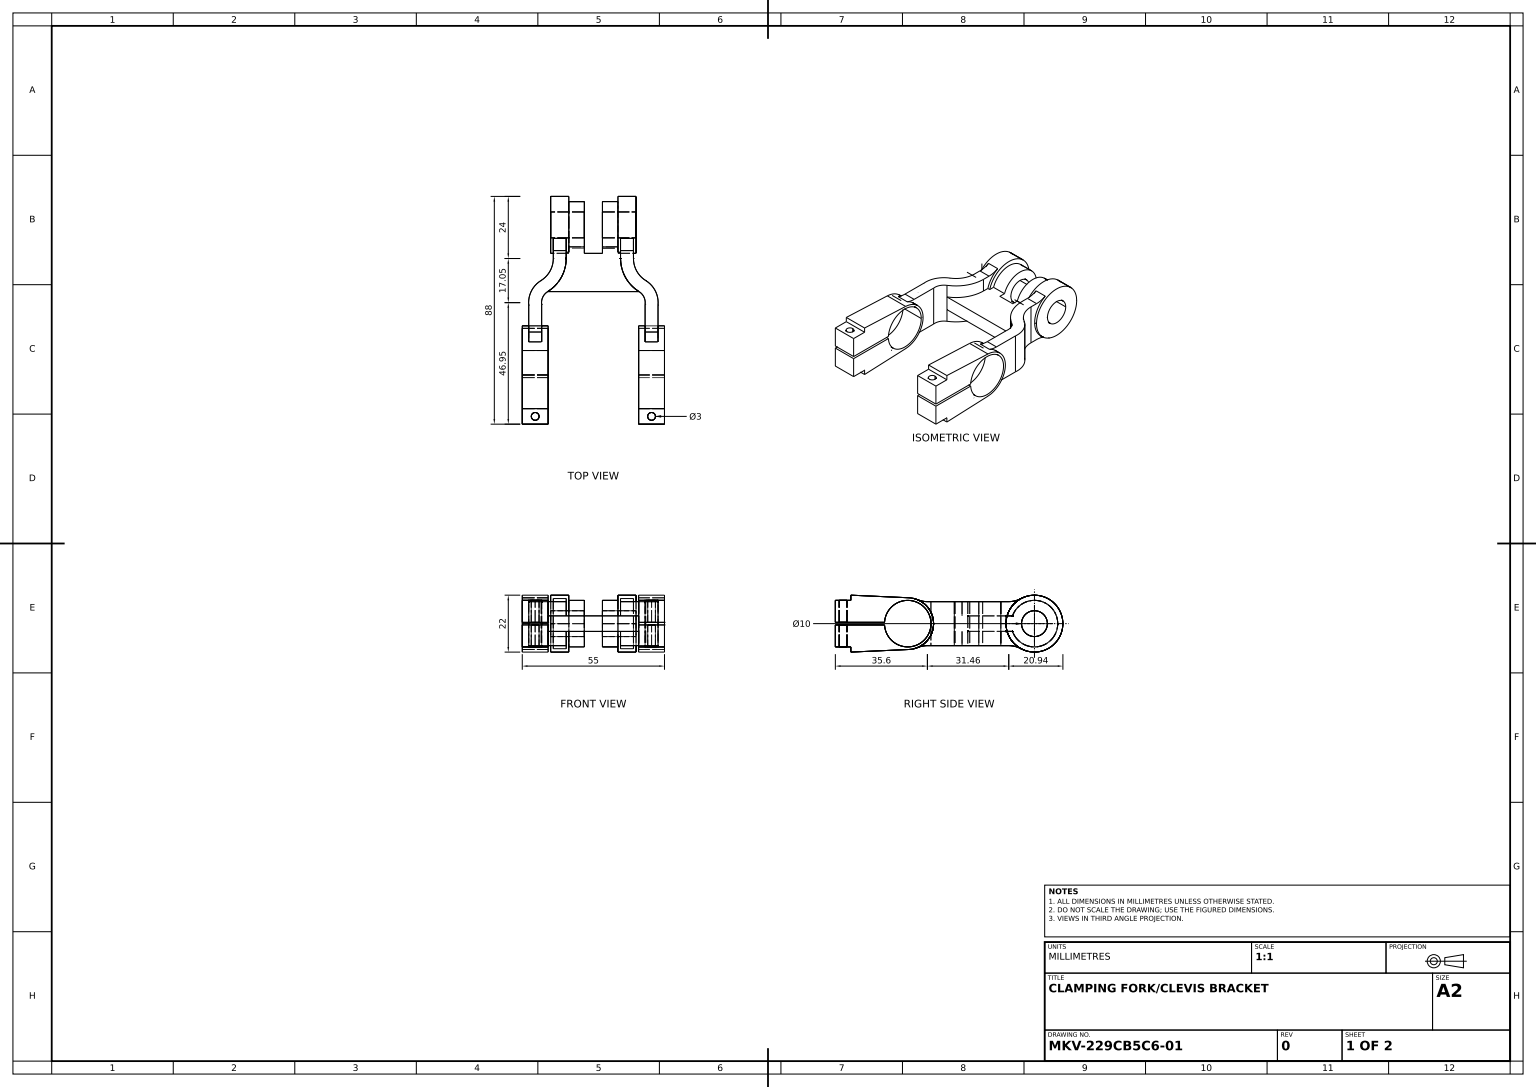
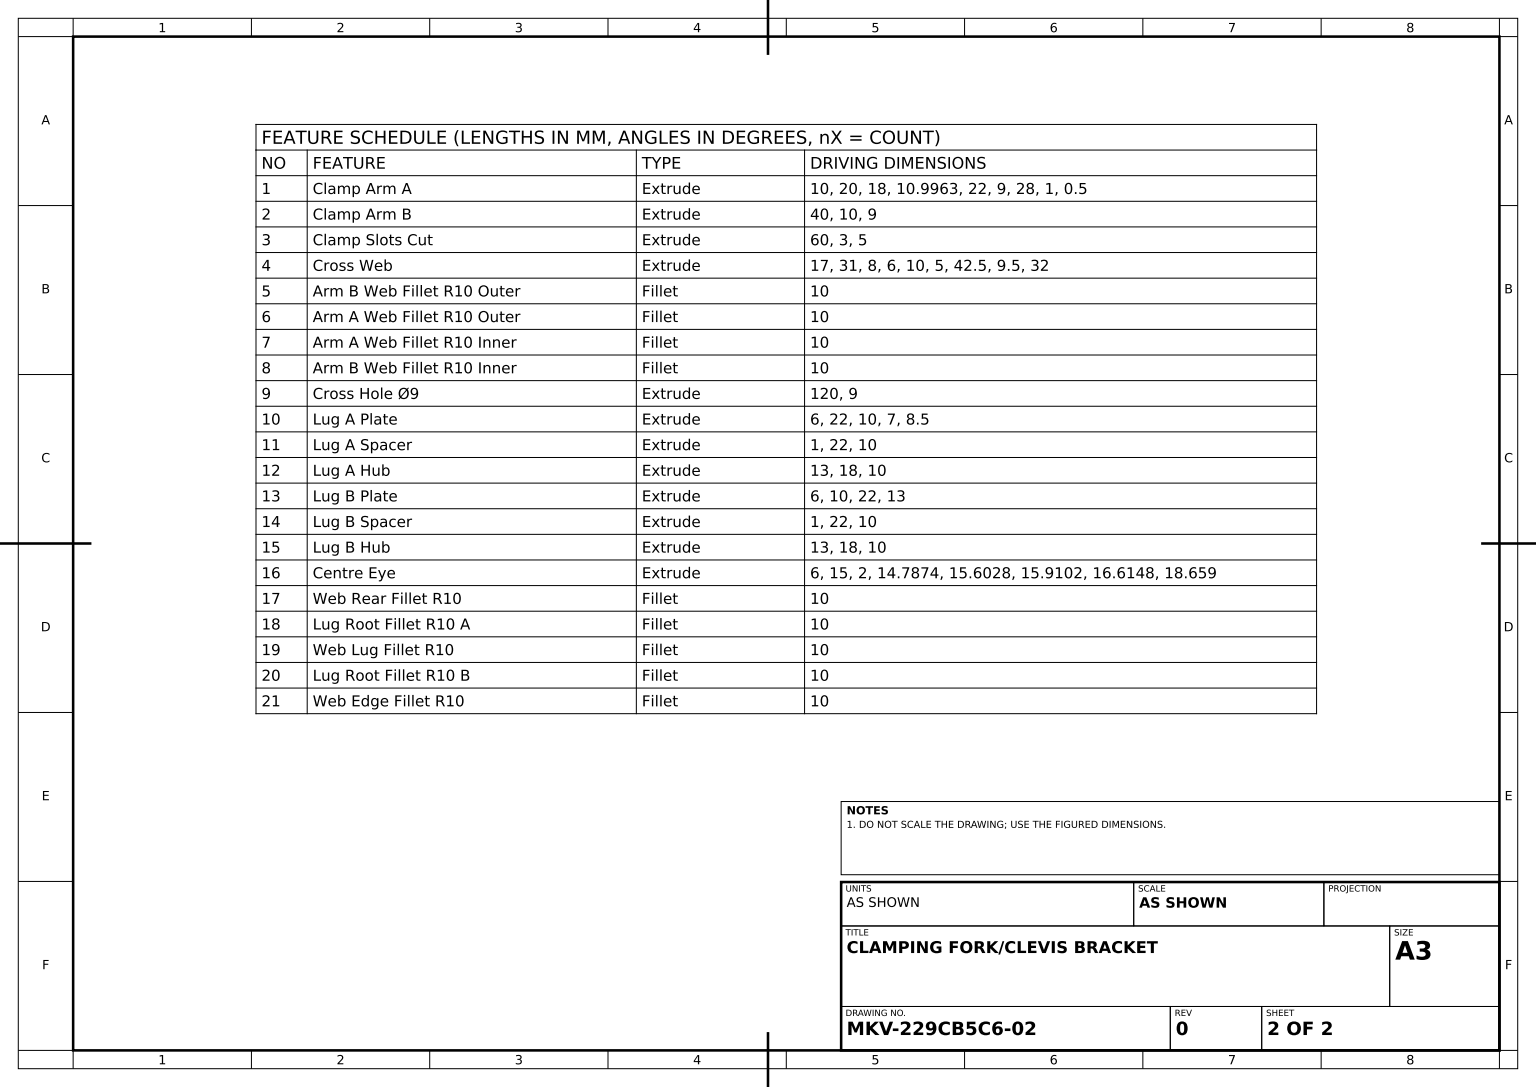
solid
v1 (-40,0.5,23.5)
v2 (-40,9,23.5)
e1 v1 v2 LINE
v3 (-40,0.5,26.5)
e2 v1 v3 CIRCLE(AX(P(-40,0.5,25),D(0,-1,0),D(0,0,-1)),1.5)
v4 (-40,9,26.5)
e3 v3 v4 LINE
e4 v4 v2 CIRCLE(AX(P(-40,9,25),D(0,1,0),D(0,0,1)),1.5)
face CYL(AX(P(-40,-51,25),D(0,1,0),D(0,0,1)),1.5) rev [-e1 e2 e3 e4]
v5 (-40,-9,23.5)
v6 (-40,-9,26.5)
e5 v5 v6 CIRCLE(AX(P(-40,-9,25),D(0,-1,0),D(0,0,-1)),1.5)
e6 v6 v5 CIRCLE(AX(P(-40,-9,25),D(0,-1,0),D(0,0,-1)),1.5)
v7 (-35,-9,28)
v8 (-35,-9,22)
e7 v7 v8 LINE
v9 (-45,-9,28)
e8 v9 v7 LINE
v10 (-45,-9,22)
e9 v9 v10 LINE
e10 v10 v8 LINE
face PLANE(AX(P(-45,-9,28),D(0,-1,0),D(0,0,-1))) [-e5 -e6] [-e7 -e8 e9 e10]
v11 (-45,-10.9962994,22)
v12 (-35,-10.9962994,22)
e11 v11 v12 LINE
e12 v8 v12 LINE
e13 v10 v11 LINE
face PLANE(AX(P(-45,-9,22),D(0,0,1),D(1,0,0))) [e11 -e12 -e10 e13]
v13 (-37.5,-9.25,-3.799671)
v14 (-37.5,0,-10)
e14 v13 v14 CIRCLE(AX(P(-37.5,0,0),D(1,0,0),D(0,0,1)),10)
v15 (-35,0,-10)
e15 v14 v15 LINE
v16 (-35,-9.9899666,-0.4478483)
e16 v16 v15 CIRCLE(AX(P(-35,0,0),D(1,0,0),D(0,0,1)),10)
v17 (-45,-9.9899666,-0.4478483)
e17 v17 v16 LINE
v18 (-45,0,-10)
e18 v17 v18 CIRCLE(AX(P(-45,0,0),D(1,0,0),D(0,0,1)),10)
v19 (-42.5,0,-10)
e19 v18 v19 LINE
v20 (-42.5,-9.25,-3.799671)
e20 v19 v20 CIRCLE(AX(P(-42.5,0,0),D(-1,0,0),D(0,0,-1)),10)
e21 v20 v13 LINE
face CYL(AX(P(-45,0,0),D(1,0,0),D(0,0,-1)),10) [e14 e15 -e16 -e17 e18 e19 e20 e21]
v21 (-1,0,-44)
v22 (-1,0,-54)
e22 v21 v22 CIRCLE(AX(P(-1,0,-49),D(1,0,0),D(0,0,-1)),5)
v23 (-14,0,-54)
e23 v23 v22 LINE
v24 (-14,0,-44)
e24 v24 v23 CIRCLE(AX(P(-14,0,-49),D(1,0,0),D(0,0,-1)),5)
e25 v24 v21 LINE
face CYL(AX(P(-8,0,-49),D(1,0,0),D(0,0,-1)),5) rev [e22 -e23 -e24 e25]
v25 (-35,0.5,8.9861004)
v26 (-35,0,-9)
e26 v25 v26 CIRCLE(AX(P(-35,0,0),D(-1,0,0),D(0,0,1)),9)
v27 (-45,0.5,8.9861004)
e27 v27 v25 LINE
v28 (-45,0,-9)
e28 v27 v28 CIRCLE(AX(P(-45,0,0),D(-1,0,0),D(0,0,1)),9)
e29 v28 v26 LINE
face CYL(AX(P(-45,0,0),D(1,0,0),D(0,0,-1)),9) rev [-e26 -e27 e28 e29]
v29 (-7,-9.6904762,-43.7947458)
v30 (-7,-8.5,-39.0626965)
e30 v29 v30 CIRCLE(AX(P(-7,-18.5,-39.0626965),D(1,0,0),D(0,0,-1)),10)
v31 (-2,-9.6904762,-43.7947458)
e31 v31 v29 LINE
v32 (-2,-8.5,-39.0626965)
e32 v32 v31 CIRCLE(AX(P(-2,-18.5,-39.0626965),D(-1,0,0),D(0,0,1)),10)
e33 v30 v32 LINE
face CYL(AX(P(-8,-18.5,-39.0626965),D(1,0,0),D(0,0,-1)),10) rev [-e30 -e31 -e32 -e33]
v33 (0.1589299,3,-23.2125992)
v34 (0.1589299,-3,-23.2125992)
e34 v33 v34 LINE
v35 (-35.1589299,3,-23.2125992)
e35 v35 v33 LINE
v36 (-35.1589299,-3,-23.2125992)
e36 v35 v36 LINE
e37 v36 v34 LINE
face PLANE(AX(P(0,3,-23.2125992),D(0,0,-1),D(-1,0,0))) rev [-e34 -e35 e36 e37]
v37 (-42.5,9.25,-3.799671)
e38 v37 v19 CIRCLE(AX(P(-42.5,0,0),D(-1,0,0),D(0,0,-1)),10)
v38 (-42.5,8.5,-7.5993421)
e39 v37 v38 CIRCLE(AX(P(-42.5,18.5,-7.5993421),D(1,0,0),D(0,0,-1)),10)
v39 (-42.5,8.5,-18)
e40 v39 v38 LINE
v40 (-42.5,-8.5,-18)
e41 v39 v40 LINE
v41 (-42.5,-8.5,-7.5993421)
e42 v40 v41 LINE
e43 v41 v20 CIRCLE(AX(P(-42.5,-18.5,-7.5993421),D(1,0,0),D(0,0,-1)),10)
face PLANE(AX(P(-42.5,8.5,-10),D(1,0,0),D(0,0,-1))) rev [-e38 e39 -e40 e41 e42 e43 -e20]
v42 (-40,-0.5,23.5)
v43 (-40,-0.5,26.5)
e44 v42 v43 CIRCLE(AX(P(-40,-0.5,25),D(0,1,0),D(0,0,1)),1.5)
e45 v43 v42 CIRCLE(AX(P(-40,-0.5,25),D(0,1,0),D(0,0,1)),1.5)
v44 (-35,-0.5,8.9861004)
v45 (-35,-0.5,28)
e46 v44 v45 LINE
v46 (-45,-0.5,8.9861004)
e47 v46 v44 LINE
v47 (-45,-0.5,28)
e48 v46 v47 LINE
e49 v47 v45 LINE
face PLANE(AX(P(-45,-0.5,8.9861004),D(0,1,0),D(0,0,1))) [-e44 -e45] [-e46 -e47 e48 e49]
v48 (2.5,9.25,-3.799671)
v49 (2.5,8.5,-7.5993421)
e50 v48 v49 CIRCLE(AX(P(2.5,18.5,-7.5993421),D(1,0,0),D(0,0,-1)),10)
v50 (2.5,8.5,-18.2790493)
e51 v50 v49 LINE
v51 (2.5,-8.5,-18.2790493)
e52 v50 v51 LINE
v52 (2.5,-8.5,-7.5993421)
e53 v51 v52 LINE
v53 (2.5,-9.25,-3.799671)
e54 v52 v53 CIRCLE(AX(P(2.5,-18.5,-7.5993421),D(1,0,0),D(0,0,-1)),10)
e55 v53 v48 CIRCLE(AX(P(2.5,0,0),D(1,0,0),D(0,0,-1)),10)
face PLANE(AX(P(2.5,8.5,-10),D(1,0,0),D(0,0,-1))) rev [e50 -e51 e52 e53 e54 e55]
v54 (5,0.5,26.5)
v55 (5,0.5,23.5)
e56 v54 v55 CIRCLE(AX(P(5,0.5,25),D(0,1,0),D(0,0,1)),1.5)
e57 v55 v54 CIRCLE(AX(P(5,0.5,25),D(0,1,0),D(0,0,1)),1.5)
v56 (10,0.5,8.9861004)
v57 (0,0.5,8.9861004)
e58 v56 v57 LINE
v58 (10,0.5,28)
e59 v58 v56 LINE
v59 (0,0.5,28)
e60 v58 v59 LINE
e61 v59 v57 LINE
face PLANE(AX(P(10,0.5,0),D(0,1,0),D(0,0,1))) rev [e56 e57] [-e58 -e59 e60 e61]
v60 (10,10.9962994,22)
v61 (0,10.9962994,22)
e62 v60 v61 LINE
v62 (0,9,22)
e63 v62 v61 LINE
v63 (10,9,22)
e64 v63 v62 LINE
e65 v63 v60 LINE
face PLANE(AX(P(10,0,22),D(0,0,1),D(1,0,0))) [e62 -e63 -e64 e65]
e66 v47 v9 LINE
e67 v45 v7 LINE
face PLANE(AX(P(-45,-0.5,28),D(0,0,1),D(0,-1,0))) [e66 e8 -e67 -e49]
v64 (-7,3,-38.4169948)
v65 (-8,3,-38.4169948)
e68 v64 v65 LINE
v66 (-8,3,-40.5147186)
e69 v66 v65 LINE
v67 (-14,3,-40.5147186)
e70 v66 v67 LINE
v68 (-14,3,-38)
e71 v68 v67 LINE
v69 (-21,3,-38)
e72 v69 v68 LINE
v70 (-21,3,-40.5147186)
e73 v70 v69 LINE
v71 (-27,3,-40.5147186)
e74 v71 v70 LINE
v72 (-27,3,-38.4169948)
e75 v72 v71 LINE
v73 (-28,3,-38.4169948)
e76 v73 v72 LINE
v74 (-28,3,-36)
e77 v74 v73 LINE
e78 v35 v74 CIRCLE(AX(P(-43,3,-36),D(0,1,0),D(0,0,1)),15)
v75 (-7,3,-36)
e79 v33 v75 CIRCLE(AX(P(8,3,-36),D(0,-1,0),D(0,0,1)),15)
e80 v64 v75 LINE
face PLANE(AX(P(0,3,0),D(0,1,0),D(0,0,1))) [e68 -e69 e70 -e71 -e72 -e73 -e74 -e75 -e76 -e77 -e78 e35 e79 -e80]
v76 (-2,0,-38)
e81 v76 v31 CIRCLE(AX(P(-2,0,-49),D(1,0,0),D(0,0,-1)),11)
v77 (-2,9.6904762,-43.7947458)
e82 v77 v76 CIRCLE(AX(P(-2,0,-49),D(1,0,0),D(0,0,-1)),11)
v78 (-2,8.5,-39.0626965)
e83 v77 v78 CIRCLE(AX(P(-2,18.5,-39.0626965),D(-1,0,0),D(0,0,1)),10)
v79 (-2,8.5,-36)
e84 v79 v78 LINE
v80 (-2,-8.5,-36)
e85 v79 v80 LINE
e86 v80 v32 LINE
face PLANE(AX(P(-2,8.5,-42),D(-1,0,0),D(0,0,1))) rev [e32 -e81 -e82 e83 -e84 e85 e86]
v81 (7.5,8.5,-7.5993421)
e87 v49 v81 LINE
v82 (7.5,9.25,-3.799671)
e88 v82 v48 LINE
e89 v81 v82 CIRCLE(AX(P(7.5,18.5,-7.5993421),D(-1,0,0),D(0,0,1)),10)
face CYL(AX(P(10,18.5,-7.5993421),D(-1,0,0),D(0,0,1)),10) rev [-e87 -e50 -e88 -e89]
v83 (-45,10.9962994,22)
v84 (-35,10.9962994,22)
e90 v83 v84 LINE
v85 (-35,9.9899666,-0.4478483)
e91 v85 v84 LINE
v86 (-45,9.9899666,-0.4478483)
e92 v86 v85 LINE
e93 v86 v83 LINE
face PLANE(AX(P(-45,9.9899666,-0.4478483),D(0,0.998996656,-0.044784834),D(0,0.044784834,0.998996656))) [e90 -e91 -e92 e93]
v87 (2.7726199,8.5,-27.4750661)
e94 v87 v79 CIRCLE(AX(P(8,8.5,-36),D(0,-1,0),D(0,0,-1)),10)
v88 (2.7726199,-8.5,-27.4750661)
e95 v87 v88 LINE
e96 v88 v80 CIRCLE(AX(P(8,-8.5,-36),D(0,-1,0),D(0,0,-1)),10)
face CYL(AX(P(8,8.5,-36),D(0,-1,0),D(0,0,-1)),10) rev [-e94 e95 e96 -e85]
v89 (7.5,-9.25,-3.799671)
e97 v53 v89 LINE
e98 v82 v89 CIRCLE(AX(P(7.5,0,0),D(-1,0,0),D(0,0,1)),10)
v90 (0,-9.9899666,-0.4478483)
v91 (0,9.9899666,-0.4478483)
e99 v90 v91 CIRCLE(AX(P(0,0,0),D(1,0,0),D(0,0,-1)),10)
v92 (10,9.9899666,-0.4478483)
e100 v92 v91 LINE
v93 (10,-9.9899666,-0.4478483)
e101 v93 v92 CIRCLE(AX(P(10,0,0),D(1,0,0),D(0,0,-1)),10)
e102 v93 v90 LINE
face CYL(AX(P(10,0,0),D(-1,0,0),D(0,0,1)),10) [e97 -e98 e88 -e55] [e99 -e100 -e101 e102]
v94 (5,-9,23.5)
v95 (5,-9,26.5)
e103 v94 v95 CIRCLE(AX(P(5,-9,25),D(0,1,0),D(0,0,1)),1.5)
v96 (5,-0.5,23.5)
e104 v94 v96 LINE
v97 (5,-0.5,26.5)
e105 v96 v97 CIRCLE(AX(P(5,-0.5,25),D(0,1,0),D(0,0,1)),1.5)
e106 v95 v97 LINE
face CYL(AX(P(5,-51,25),D(0,1,0),D(0,0,1)),1.5) rev [-e103 e104 e105 -e106]
e107 v15 v85 CIRCLE(AX(P(-35,0,0),D(1,0,0),D(0,0,1)),10)
v98 (-35,9,22)
e108 v84 v98 LINE
v99 (-35,9,28)
e109 v98 v99 LINE
v100 (-35,0.5,28)
e110 v99 v100 LINE
e111 v100 v25 LINE
e112 v26 v44 CIRCLE(AX(P(-35,0,0),D(-1,0,0),D(0,0,1)),9)
e113 v12 v16 LINE
face PLANE(AX(P(-35,0,0),D(-1,0,0),D(0,0,1))) rev [e107 e91 e108 e109 e110 e111 e26 e112 e46 e67 e7 e12 e113 e16]
v101 (-7,9.6904762,-43.7947458)
e114 v101 v64 CIRCLE(AX(P(-7,0,-49),D(1,0,0),D(0,0,-1)),11)
v102 (-7,8.5,-36)
e115 v102 v75 LINE
v103 (-7,8.5,-39.0626965)
e116 v103 v102 LINE
e117 v103 v101 CIRCLE(AX(P(-7,18.5,-39.0626965),D(1,0,0),D(0,0,-1)),10)
face PLANE(AX(P(-7,8.5,-42),D(1,0,0),D(0,0,-1))) rev [e114 e80 -e115 -e116 e117]
v104 (-1,0,-38)
e118 v76 v104 LINE
v105 (-1,0,-60)
e119 v105 v104 CIRCLE(AX(P(-1,0,-49),D(1,0,0),D(0,0,-1)),11)
v106 (-8,0,-60)
e120 v106 v105 LINE
e121 v106 v65 CIRCLE(AX(P(-8,0,-49),D(1,0,0),D(0,0,-1)),11)
e122 v101 v77 LINE
face CYL(AX(P(-8,0,-49),D(1,0,0),D(0,0,-1)),11) [e118 -e119 -e120 e121 -e68 -e114 e122 e82]
v107 (-45,0.5,28)
e123 v107 v100 LINE
e124 v107 v27 LINE
e125 v3 v1 CIRCLE(AX(P(-40,0.5,25),D(0,-1,0),D(0,0,-1)),1.5)
face PLANE(AX(P(-45,0.5,28),D(0,-1,0),D(0,0,-1))) [e27 -e111 -e123 e124] [-e125 -e2]
v108 (10,-10.9962994,22)
e126 v108 v93 LINE
e127 v60 v92 LINE
v109 (10,9,28)
e128 v109 v63 LINE
e129 v58 v109 LINE
v110 (10,-0.5,8.9861004)
e130 v110 v56 CIRCLE(AX(P(10,0,0),D(1,0,0),D(0,0,-1)),9)
v111 (10,-0.5,28)
e131 v111 v110 LINE
v112 (10,-9,28)
e132 v112 v111 LINE
v113 (10,-9,22)
e133 v112 v113 LINE
e134 v108 v113 LINE
face PLANE(AX(P(10,0,0),D(1,0,0),D(0,0,-1))) [e126 e101 -e127 -e65 -e128 -e129 e59 -e130 -e131 -e132 e133 -e134]
v114 (-8,-3,-40.5147186)
v115 (-8,0,-58)
e135 v114 v115 CIRCLE(AX(P(-8,0,-49),D(1,0,0),D(0,0,-1)),9)
e136 v115 v66 CIRCLE(AX(P(-8,0,-49),D(1,0,0),D(0,0,-1)),9)
v116 (-8,-3,-38.4169948)
e137 v116 v106 CIRCLE(AX(P(-8,0,-49),D(1,0,0),D(0,0,-1)),11)
e138 v114 v116 LINE
face PLANE(AX(P(-8,0,-49),D(1,0,0),D(0,0,-1))) rev [e135 e136 e69 -e121 -e137 -e138]
v117 (0.1589299,8.5,-23.2125992)
e139 v117 v33 LINE
e140 v102 v117 CIRCLE(AX(P(8,8.5,-36),D(0,1,0),D(0,0,-1)),15)
face CYL(AX(P(8,8.5,-36),D(0,-1,0),D(0,0,-1)),15) [-e139 -e140 e115 -e79]
v118 (0,-10.9962994,22)
e141 v108 v118 LINE
e142 v118 v90 LINE
face PLANE(AX(P(10,-9.9899666,-0.4478483),D(0,0.998996656,0.044784834),D(0,-0.044784834,0.998996656))) rev [-e102 -e126 e141 e142]
e143 v117 v50 CIRCLE(AX(P(-2.4547601,8.5,-18.9501322),D(0,-1,0),D(0,0,1)),5)
v119 (7.5,8.5,-18)
e144 v81 v119 LINE
e145 v119 v87 CIRCLE(AX(P(-2.4547601,8.5,-18.9501322),D(0,1,0),D(0,0,1)),10)
e146 v78 v103 LINE
face PLANE(AX(P(8,8.5,-36),D(0,-1,0),D(0,0,-1))) rev [e140 e143 e51 e87 e144 e145 e94 e84 e146 e116]
v120 (-45,9,28)
e147 v120 v107 LINE
e148 v120 v99 LINE
face PLANE(AX(P(-45,9,28),D(0,0,1),D(1,0,0))) [e147 e123 -e110 -e148]
e149 v5 v42 LINE
e150 v6 v43 LINE
face CYL(AX(P(-40,-51,25),D(0,1,0),D(0,0,1)),1.5) rev [-e149 e5 e150 e45]
e151 v2 v4 CIRCLE(AX(P(-40,9,25),D(0,1,0),D(0,0,1)),1.5)
face CYL(AX(P(-40,-51,25),D(0,1,0),D(0,0,1)),1.5) rev [e151 -e3 e125 e1]
v121 (-7,-3,-38.4169948)
e152 v121 v29 CIRCLE(AX(P(-7,0,-49),D(1,0,0),D(0,0,-1)),11)
v122 (-7,-8.5,-36)
e153 v30 v122 LINE
v123 (-7,-3,-36)
e154 v123 v122 LINE
e155 v121 v123 LINE
face PLANE(AX(P(-7,8.5,-42),D(1,0,0),D(0,0,-1))) rev [e152 e30 e153 -e154 -e155]
v124 (-21,-3,-38)
e156 v69 v124 LINE
v125 (-21,-3,-40.5147186)
e157 v125 v124 LINE
e158 v70 v125 CIRCLE(AX(P(-21,0,-49),D(-1,0,0),D(0,0,1)),9)
v126 (-21,0,-44)
v127 (-21,0,-54)
e159 v126 v127 CIRCLE(AX(P(-21,0,-49),D(-1,0,0),D(0,0,1)),5)
e160 v127 v126 CIRCLE(AX(P(-21,0,-49),D(-1,0,0),D(0,0,1)),5)
face PLANE(AX(P(-21,3,0),D(1,0,0),D(0,0,-1))) [e156 -e157 -e158 e73] [e159 e160]
v128 (5,9,23.5)
e161 v55 v128 LINE
v129 (5,9,26.5)
e162 v128 v129 CIRCLE(AX(P(5,9,25),D(0,1,0),D(0,0,1)),1.5)
e163 v54 v129 LINE
face CYL(AX(P(5,-51,25),D(0,1,0),D(0,0,1)),1.5) rev [e161 e162 -e163 -e57]
e164 v11 v17 LINE
face PLANE(AX(P(-45,-10.9962994,22),D(0,-0.998996656,-0.044784834),D(0,0.044784834,-0.998996656))) [e164 e17 -e113 -e11]
v130 (-34,0,-54)
e165 v127 v130 LINE
v131 (-34,0,-44)
e166 v130 v131 CIRCLE(AX(P(-34,0,-49),D(-1,0,0),D(0,0,1)),5)
e167 v126 v131 LINE
face CYL(AX(P(-27,0,-49),D(-1,0,0),D(0,0,1)),5) rev [e165 e166 -e167 -e160]
v132 (-37.5,8.5,-18.2790493)
v133 (-35.1589299,8.5,-23.2125992)
e168 v132 v133 CIRCLE(AX(P(-32.5452399,8.5,-18.9501322),D(0,-1,0),D(0,0,-1)),5)
v134 (-37.5,-8.5,-18.2790493)
e169 v132 v134 LINE
v135 (-35.1589299,-8.5,-23.2125992)
e170 v134 v135 CIRCLE(AX(P(-32.5452399,-8.5,-18.9501322),D(0,-1,0),D(0,0,-1)),5)
e171 v36 v135 LINE
e172 v133 v35 LINE
face CYL(AX(P(-32.5452399,8.5,-18.9501322),D(0,-1,0),D(0,0,-1)),5) rev [-e168 e169 e170 -e171 -e36 -e172]
v136 (-28,-3,-38.4169948)
v137 (-27,-3,-38.4169948)
e173 v136 v137 LINE
v138 (-28,-9.6904762,-43.7947458)
e174 v138 v136 CIRCLE(AX(P(-28,0,-49),D(-1,0,0),D(0,0,1)),11)
v139 (-33,-9.6904762,-43.7947458)
e175 v138 v139 LINE
v140 (-33,0,-38)
e176 v139 v140 CIRCLE(AX(P(-33,0,-49),D(-1,0,0),D(0,0,1)),11)
v141 (-34,0,-38)
e177 v140 v141 LINE
v142 (-34,0,-60)
e178 v142 v141 CIRCLE(AX(P(-34,0,-49),D(-1,0,0),D(0,0,1)),11)
v143 (-27,0,-60)
e179 v143 v142 LINE
e180 v143 v137 CIRCLE(AX(P(-27,0,-49),D(-1,0,0),D(0,0,1)),11)
face CYL(AX(P(-27,0,-49),D(-1,0,0),D(0,0,1)),11) [-e173 -e174 e175 e176 e177 -e178 -e179 e180]
v144 (-27,-3,-40.5147186)
e181 v144 v125 LINE
e182 v71 v144 CIRCLE(AX(P(-27,0,-49),D(-1,0,0),D(0,0,1)),9)
face CYL(AX(P(-21,0,-49),D(-1,0,0),D(0,0,1)),9) [-e181 -e182 e74 e158]
v145 (-33,-8.5,-39.0626965)
e183 v139 v145 CIRCLE(AX(P(-33,-18.5,-39.0626965),D(1,0,0),D(0,0,-1)),10)
v146 (-28,-8.5,-39.0626965)
e184 v146 v138 CIRCLE(AX(P(-28,-18.5,-39.0626965),D(-1,0,0),D(0,0,1)),10)
e185 v145 v146 LINE
face CYL(AX(P(-27,-18.5,-39.0626965),D(-1,0,0),D(0,0,1)),10) rev [-e183 -e175 -e184 -e185]
v147 (-37.5,9.25,-3.799671)
e186 v147 v37 LINE
v148 (-37.5,8.5,-7.5993421)
e187 v148 v147 CIRCLE(AX(P(-37.5,18.5,-7.5993421),D(-1,0,0),D(0,0,1)),10)
e188 v38 v148 LINE
face CYL(AX(P(-45,18.5,-7.5993421),D(1,0,0),D(0,0,-1)),10) rev [-e186 -e187 -e188 -e39]
v149 (-45,9,22)
e189 v149 v98 LINE
e190 v149 v120 LINE
face PLANE(AX(P(-45,9,22),D(0,1,0),D(0,0,1))) [-e151 -e4] [-e189 e190 e148 -e109]
v150 (0.1589299,-8.5,-23.2125992)
e191 v34 v150 LINE
e192 v150 v51 CIRCLE(AX(P(-2.4547601,-8.5,-18.9501322),D(0,-1,0),D(0,0,1)),5)
face CYL(AX(P(-2.4547601,8.5,-18.9501322),D(0,-1,0),D(0,0,-1)),5) rev [e34 e191 e192 -e52 -e143 e139]
face CYL(AX(P(-40,-51,25),D(0,1,0),D(0,0,1)),1.5) rev [e44 -e150 e6 e149]
e193 v14 v147 CIRCLE(AX(P(-37.5,0,0),D(1,0,0),D(0,0,1)),10)
v151 (-37.5,-8.5,-7.5993421)
e194 v13 v151 CIRCLE(AX(P(-37.5,-18.5,-7.5993421),D(-1,0,0),D(0,0,1)),10)
e195 v151 v134 LINE
e196 v148 v132 LINE
face PLANE(AX(P(-37.5,8.5,-10),D(-1,0,0),D(0,0,1))) rev [e187 -e193 -e14 e194 e195 -e169 -e196]
v152 (-14,-3,-38)
v153 (-14,-3,-40.5147186)
e197 v152 v153 LINE
e198 v114 v153 LINE
e199 v121 v116 LINE
e200 v34 v123 CIRCLE(AX(P(8,-3,-36),D(0,-1,0),D(0,0,1)),15)
v154 (-28,-3,-36)
e201 v36 v154 CIRCLE(AX(P(-43,-3,-36),D(0,1,0),D(0,0,1)),15)
e202 v154 v136 LINE
e203 v137 v144 LINE
e204 v124 v152 LINE
face PLANE(AX(P(0,-3,0),D(0,1,0),D(0,0,1))) rev [e197 -e198 e138 -e199 e155 -e200 -e37 e201 e202 e173 e203 e181 e157 e204]
v155 (7.5,-8.5,-7.5993421)
e205 v89 v155 CIRCLE(AX(P(7.5,-18.5,-7.5993421),D(-1,0,0),D(0,0,1)),10)
v156 (7.5,-8.5,-18)
e206 v155 v156 LINE
e207 v119 v156 LINE
face PLANE(AX(P(7.5,8.5,-10),D(-1,0,0),D(0,0,1))) rev [e205 e206 -e207 -e144 e89 e98]
face CYL(AX(P(-8,18.5,-39.0626965),D(1,0,0),D(0,0,-1)),10) rev [-e117 -e146 -e83 -e122]
v157 (-37.7726199,8.5,-27.4750661)
e208 v157 v39 CIRCLE(AX(P(-32.5452399,8.5,-18.9501322),D(0,1,0),D(0,0,-1)),10)
v158 (-37.7726199,-8.5,-27.4750661)
e209 v157 v158 LINE
e210 v158 v40 CIRCLE(AX(P(-32.5452399,-8.5,-18.9501322),D(0,1,0),D(0,0,-1)),10)
face CYL(AX(P(-32.5452399,8.5,-18.9501322),D(0,-1,0),D(0,0,-1)),10) [-e41 -e208 e209 e210]
v159 (-28,9.6904762,-43.7947458)
v160 (-28,8.5,-39.0626965)
e211 v159 v160 CIRCLE(AX(P(-28,18.5,-39.0626965),D(-1,0,0),D(0,0,1)),10)
v161 (-33,9.6904762,-43.7947458)
e212 v161 v159 LINE
v162 (-33,8.5,-39.0626965)
e213 v162 v161 CIRCLE(AX(P(-33,18.5,-39.0626965),D(1,0,0),D(0,0,-1)),10)
e214 v160 v162 LINE
face CYL(AX(P(-27,18.5,-39.0626965),D(-1,0,0),D(0,0,1)),10) rev [-e211 -e212 -e213 -e214]
e215 v129 v128 CIRCLE(AX(P(5,9,25),D(0,1,0),D(0,0,1)),1.5)
face CYL(AX(P(5,-51,25),D(0,1,0),D(0,0,1)),1.5) rev [-e161 -e56 e163 e215]
e216 v151 v41 LINE
face CYL(AX(P(-45,-18.5,-7.5993421),D(1,0,0),D(0,0,-1)),10) rev [-e216 -e194 -e21 -e43]
v163 (-14,0,-58)
e217 v153 v163 CIRCLE(AX(P(-14,0,-49),D(1,0,0),D(0,0,-1)),9)
e218 v68 v152 LINE
e219 v163 v67 CIRCLE(AX(P(-14,0,-49),D(1,0,0),D(0,0,-1)),9)
e220 v23 v24 CIRCLE(AX(P(-14,0,-49),D(1,0,0),D(0,0,-1)),5)
face PLANE(AX(P(-14,0,-49),D(1,0,0),D(0,0,-1))) rev [-e217 -e197 -e218 e71 -e219] [e24 e220]
e221 v18 v86 CIRCLE(AX(P(-45,0,0),D(1,0,0),D(0,0,1)),10)
face CYL(AX(P(-45,0,0),D(1,0,0),D(0,0,-1)),10) [e221 e92 -e107 -e15 e193 e186 e38 -e19]
v164 (-28,-8.5,-36)
e222 v135 v164 CIRCLE(AX(P(-43,-8.5,-36),D(0,1,0),D(0,0,1)),15)
e223 v154 v164 LINE
face CYL(AX(P(-43,8.5,-36),D(0,-1,0),D(0,0,-1)),15) [e222 -e223 -e201 e171]
v165 (-28,8.5,-36)
e224 v165 v74 LINE
e225 v133 v165 CIRCLE(AX(P(-43,8.5,-36),D(0,1,0),D(0,0,1)),15)
face CYL(AX(P(-43,8.5,-36),D(0,-1,0),D(0,0,-1)),15) [e78 -e224 -e225 e172]
v166 (0,-9,22)
e226 v113 v166 LINE
e227 v118 v166 LINE
face PLANE(AX(P(10,0,22),D(0,0,1),D(1,0,0))) [-e141 e134 e226 -e227]
e228 v22 v21 CIRCLE(AX(P(-1,0,-49),D(1,0,0),D(0,0,-1)),5)
face CYL(AX(P(-8,0,-49),D(1,0,0),D(0,0,-1)),5) rev [-e25 -e220 e23 e228]
e229 v122 v150 CIRCLE(AX(P(8,-8.5,-36),D(0,1,0),D(0,0,-1)),15)
face CYL(AX(P(8,8.5,-36),D(0,-1,0),D(0,0,-1)),15) [e154 e229 -e191 e200]
e230 v72 v143 CIRCLE(AX(P(-27,0,-49),D(-1,0,0),D(0,0,1)),11)
face PLANE(AX(P(-27,0,-49),D(-1,0,0),D(0,0,1))) rev [-e203 -e180 -e230 e75 e182]
e231 v28 v46 CIRCLE(AX(P(-45,0,0),D(-1,0,0),D(0,0,1)),9)
e232 v83 v149 LINE
face PLANE(AX(P(-45,0,0),D(-1,0,0),D(0,0,1))) [-e93 -e221 -e18 -e164 -e13 -e9 -e66 -e48 -e231 -e28 -e124 -e147 -e190 -e232]
e233 v163 v115 LINE
face CYL(AX(P(-14,0,-49),D(1,0,0),D(0,0,-1)),9) [e198 e217 e233 -e135]
e234 v164 v146 LINE
face PLANE(AX(P(-28,8.5,-42),D(-1,0,0),D(0,0,1))) rev [e184 e174 -e202 e223 e234]
e235 v61 v91 LINE
v167 (0,-9,28)
e236 v167 v166 LINE
v168 (0,-0.5,28)
e237 v167 v168 LINE
v169 (0,-0.5,8.9861004)
e238 v168 v169 LINE
e239 v169 v57 CIRCLE(AX(P(0,0,0),D(1,0,0),D(0,0,-1)),9)
v170 (0,9,28)
e240 v59 v170 LINE
e241 v170 v62 LINE
face PLANE(AX(P(0,0,0),D(1,0,0),D(0,0,-1))) rev [e235 -e99 -e142 e227 -e236 e237 e238 e239 -e61 e240 e241 e63]
e242 v104 v105 CIRCLE(AX(P(-1,0,-49),D(1,0,0),D(0,0,-1)),11)
face CYL(AX(P(-8,0,-49),D(1,0,0),D(0,0,-1)),11) [-e118 e81 e31 -e152 e199 e137 e120 -e242]
face CYL(AX(P(-14,0,-49),D(1,0,0),D(0,0,-1)),9) [-e70 -e136 -e233 e219]
e243 v141 v142 CIRCLE(AX(P(-34,0,-49),D(-1,0,0),D(0,0,1)),11)
e244 v140 v161 CIRCLE(AX(P(-33,0,-49),D(-1,0,0),D(0,0,1)),11)
e245 v73 v159 CIRCLE(AX(P(-28,0,-49),D(-1,0,0),D(0,0,1)),11)
face CYL(AX(P(-27,0,-49),D(-1,0,0),D(0,0,1)),11) [e179 -e243 -e177 e244 e212 -e245 e76 e230]
v171 (-33,-8.5,-36)
e246 v145 v171 LINE
e247 v171 v158 CIRCLE(AX(P(-43,-8.5,-36),D(0,-1,0),D(0,0,1)),10)
face PLANE(AX(P(-32.5452399,-8.5,-18.9501322),D(0,-1,0),D(0,0,-1))) [-e246 e185 -e234 -e222 -e170 -e195 e216 -e42 -e210 -e247]
e248 v156 v88 CIRCLE(AX(P(-2.4547601,-8.5,-18.9501322),D(0,1,0),D(0,0,1)),10)
face CYL(AX(P(-2.4547601,8.5,-18.9501322),D(0,-1,0),D(0,0,-1)),10) [-e95 -e145 e207 e248]
e249 v110 v169 LINE
face CYL(AX(P(10,0,0),D(-1,0,0),D(0,0,1)),9) rev [-e239 -e249 e130 e58]
e250 v165 v160 LINE
v172 (-33,8.5,-36)
e251 v162 v172 LINE
e252 v172 v157 CIRCLE(AX(P(-43,8.5,-36),D(0,-1,0),D(0,0,1)),10)
face PLANE(AX(P(-32.5452399,8.5,-18.9501322),D(0,-1,0),D(0,0,-1))) rev [e250 e214 e251 e252 e208 e40 e188 e196 e168 e225]
face PLANE(AX(P(-1,0,-49),D(1,0,0),D(0,0,-1))) [e242 e119] [-e228 -e22]
e253 v131 v130 CIRCLE(AX(P(-34,0,-49),D(-1,0,0),D(0,0,1)),5)
face PLANE(AX(P(-34,0,-49),D(-1,0,0),D(0,0,1))) [-e253 -e166] [e243 e178]
e254 v155 v52 LINE
face CYL(AX(P(10,-18.5,-7.5993421),D(-1,0,0),D(0,0,1)),10) rev [-e254 -e205 -e97 -e54]
face PLANE(AX(P(-45,10.9962994,22),D(0,0,1),D(1,0,0))) [e232 e189 -e108 -e90]
e255 v109 v170 LINE
face PLANE(AX(P(10,0,28),D(0,0,1),D(1,0,0))) [e255 -e240 -e60 e129]
face CYL(AX(P(-27,0,-49),D(-1,0,0),D(0,0,1)),5) rev [e167 e253 -e165 -e159]
e256 v97 v96 CIRCLE(AX(P(5,-0.5,25),D(0,1,0),D(0,0,1)),1.5)
e257 v95 v94 CIRCLE(AX(P(5,-9,25),D(0,1,0),D(0,0,1)),1.5)
face CYL(AX(P(5,-51,25),D(0,1,0),D(0,0,1)),1.5) rev [e106 e256 -e104 -e257]
e258 v111 v168 LINE
face PLANE(AX(P(10,-0.5,0),D(0,1,0),D(0,0,1))) [e131 e249 -e238 -e258] [-e105 -e256]
face PLANE(AX(P(8,-8.5,-36),D(0,-1,0),D(0,0,-1))) [-e192 -e229 -e153 e33 -e86 -e96 -e248 -e206 e254 -e53]
face PLANE(AX(P(0,3,-38),D(0,0,-1),D(-1,0,0))) [e72 e218 -e204 -e156]
e259 v172 v171 LINE
face CYL(AX(P(-43,8.5,-36),D(0,-1,0),D(0,0,-1)),10) rev [-e252 e259 e247 -e209]
face PLANE(AX(P(-28,8.5,-42),D(-1,0,0),D(0,0,1))) rev [e224 e77 e245 e211 -e250]
e260 v112 v167 LINE
face PLANE(AX(P(10,-9,0),D(0,1,0),D(0,0,1))) rev [e260 e236 -e226 -e133] [e257 e103]
face PLANE(AX(P(10,0,28),D(0,0,1),D(0,-1,0))) [e132 e258 -e237 -e260]
face PLANE(AX(P(10,9,0),D(0,1,0),D(0,0,1))) [e64 -e241 -e255 e128] [-e162 -e215]
face PLANE(AX(P(10,9.9899666,-0.4478483),D(0,0.998996656,-0.044784834),D(0,0.044784834,0.998996656))) [e127 e100 -e235 -e62]
face CYL(AX(P(-45,0,0),D(1,0,0),D(0,0,-1)),9) rev [e231 e47 -e112 -e29]
face PLANE(AX(P(-33,8.5,-42),D(1,0,0),D(0,0,-1))) rev [e213 -e244 -e176 e183 e246 -e259 -e251]
